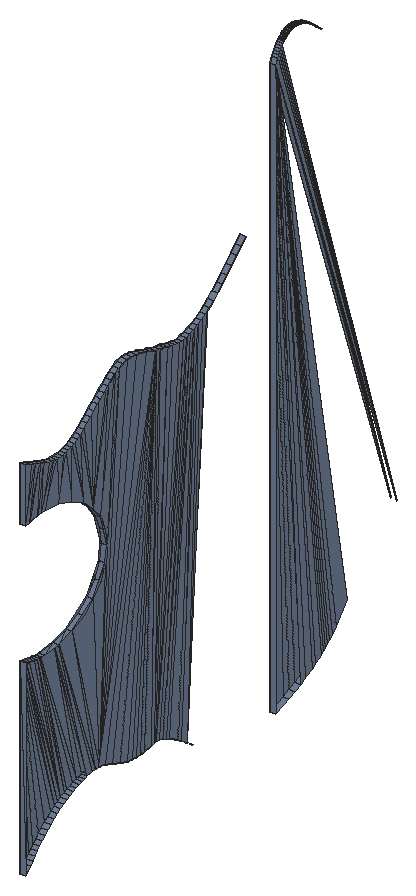
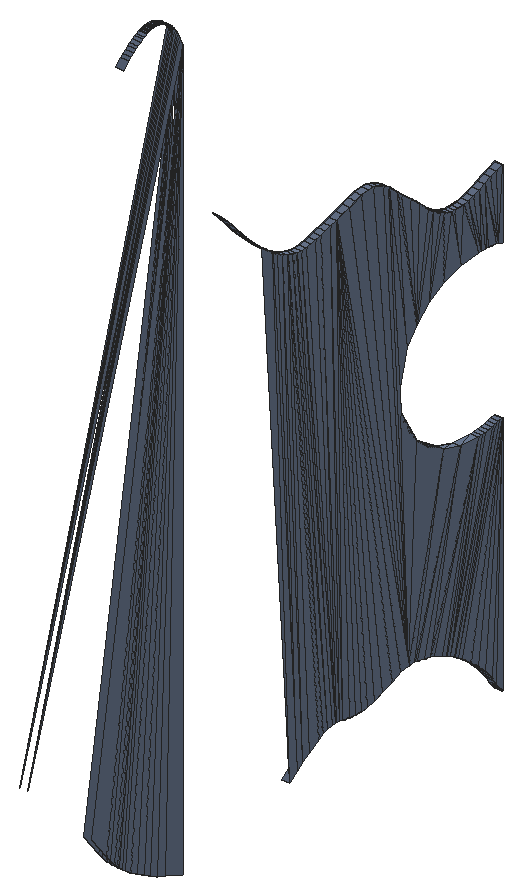
# SketchUp Ruby script. Lengths in inches.
U = 1.inch
M = Sketchup.active_model
def pt(a) = Geom::Point3d.new(a.map { |v| v * U })
def face(e, loops, mat)
  f = e.add_face(loops[0].map { |a| pt(a) })
  loops[1..].each { |l| e.add_face(l.map { |a| pt(a) }).erase! }
  f.material = f.back_material = mat if mat
  f
end
# faces: each face lists its corners as indices into pts; further lists are holes
def faces(e, pts, list, mat = nil) = list.each { |f| face(e, (f[0].is_a?(Array) ? f : [f]).map { |l| l.map { |i| pts[i] } }, mat) }
# xy, xz, yz: faces in a plane at the given z, y or x. An outline is a flat list of corners, or four numbers for a rectangle; further outlines are holes
def ring(l) = l.size == 4 ? [[l[0], l[1]], [l[2], l[1]], [l[2], l[3]], [l[0], l[3]]] : l.each_slice(2).to_a
def flat(e, list, mat, &to3) = list.each { |f| face(e, (f[0].is_a?(Array) ? f : [f]).map { |l| ring(l).map { |u, v| to3.(u, v) } }, mat) }
def xy(e, z, list, mat = nil) = flat(e, list, mat) { |x, y| [x, y, z] }
def xz(e, y, list, mat = nil) = flat(e, list, mat) { |x, z| [x, y, z] }
def yz(e, x, list, mat = nil) = flat(e, list, mat) { |y, z| [x, y, z] }
def lines(e, pts, list) = list.each { |a, b| e.add_line(pt(pts[a]), pt(pts[b])) }
# prism: a flat outline (further loops are holes) pulled along v
def prism(e, loops, v, mat = nil)
  f = face(e, loops, mat); d = Geom::Vector3d.new(v.map { |x| x * U })
  f.pushpull(f.normal.samedirection?(d) ? d.length : -d.length)
end
def box(e, o, s, mat = nil) = prism(e, [[o, [o[0] + s[0], o[1], o[2]], [o[0] + s[0], o[1] + s[1], o[2]], [o[0], o[1] + s[1], o[2]]]], [0, 0, s[2]], mat)
def at(x, y, z, deg = 0) = Geom::Transformation.translation(pt([x, y, z])) * Geom::Transformation.rotation(ORIGIN, Z_AXIS, deg.degrees)
def axes(o, x, y, z) = Geom::Transformation.new([*x, 0, *y, 0, *z, 0, *pt(o).to_a, 1])
def part(name) = M.definitions.add(name)
# library, detail: a bought-in or finely detailed component or shape, given as its bounding box
def library(name, o, s) = part(name).tap { |d| box(d.entities, o, s) }
def detail(e, o, s) = box(e.add_group.entities, o, s)
def put(e, d, t, mat = nil) = e.add_instance(d, t).tap { |i| i.material = mat if mat }
def group(e, t, mat = nil) = e.add_group.tap { |g| g.transformation = t; g.material = mat if mat }.entities
root = M.entities
M.materials.add("3D66_SU_1584934530605_002").color = [112, 126, 151]
xy(root,50.943,[[122.497,228.886,123.073,229.12]],"3D66_SU_1584934530605_002")
xz(root,216.339,[[122.497,46.745,123.073,46.745,122.497,64.189],[123.073,46.745,123.073,64.189,122.497,64.189],[122.497,75.394,123.073,80.381]],"3D66_SU_1584934530605_002")
xz(root,244.866,[[122.497,47.514,123.073,100.534]],"3D66_SU_1584934530605_002")
yz(root,122.497,[[216.339,46.745,216.339,64.189,216.821,47.359],[216.339,46.745,216.821,47.359,216.584,47.051],[216.821,47.359,216.339,64.189,217.294,47.975],[216.821,47.359,217.294,47.975,217.055,47.668],[244.866,47.514,244.866,100.534,246.341,48.072],
  [217.294,47.975,216.339,64.189,217.809,48.58],[217.294,47.975,217.809,48.58,217.543,48.28],[246.341,48.072,244.866,100.534,247.028,48.369],[247.028,48.369,244.866,100.534,247.682,48.677],[217.809,48.58,216.339,64.189,218.416,49.169],
  [217.809,48.58,218.416,49.169,218.099,48.874],[247.682,48.677,244.866,100.534,248.302,48.997],[248.302,48.997,244.866,100.534,248.888,49.328],[218.416,49.169,216.339,64.189,219.117,49.767],[218.416,49.169,219.117,49.767,218.758,49.469],
  [235.314,49.199,234.68,49.635,236.828,83.746],[235.314,49.199,236.828,83.746,237.763,84.427],[248.888,49.328,244.866,100.534,249.441,49.671],[234.68,49.635,234.12,50.01,235.941,83.225],[234.68,49.635,235.941,83.225,236.38,83.465],
  [234.68,49.635,236.38,83.465,236.828,83.746],[249.441,49.671,244.866,100.534,249.961,50.026],[219.117,49.767,216.339,64.189,219.858,50.331],[219.117,49.767,219.858,50.331,219.486,50.056],[234.12,50.01,233.621,50.329,235.506,83.026],
  [234.12,50.01,235.506,83.026,235.941,83.225],[249.961,50.026,244.866,100.534,250.206,50.211],[250.206,50.211,244.866,100.534,250.441,50.403],[233.621,50.329,232.746,50.819,235.506,83.026],[233.621,50.329,233.168,50.597,232.746,50.819],
  [219.858,50.331,216.339,64.189,220.227,50.584],[250.441,50.403,244.866,100.534,250.665,50.602],[220.227,50.584,216.339,64.189,216.63,64.114],[220.227,50.584,216.63,64.114,220.586,50.809],[250.665,50.602,244.866,100.534,250.879,50.807],
  [250.879,50.807,244.866,100.534,251.28,51.228],[220.586,50.809,216.63,64.114,216.925,64.049],[220.586,50.809,216.925,64.049,220.939,51.006],[232.746,50.819,232.342,50.998,235.506,83.026],[228.886,50.943,228.408,50.975,231.095,83.28],
  [228.886,50.943,228.653,50.952,228.408,50.975],[228.886,50.943,229.369,50.948,229.12,50.943],[228.886,50.943,231.095,83.28,229.369,50.948],[229.369,50.948,229.9375,50.983,229.644,50.954],[229.369,50.948,231.095,83.28,229.9375,50.983],
  [228.408,50.975,227.831,51.075,231.095,83.28],[228.408,50.975,228.139,51.014,227.831,51.075],[229.9375,50.983,230.538,51.124,230.234,51.047],[229.9375,50.983,231.095,83.28,230.538,51.124],[232.342,50.998,231.94,51.141,235.072,82.87],
  [232.342,50.998,235.072,82.87,235.506,83.026],[220.939,51.006,216.925,64.049,217.225,63.994],[220.939,51.006,217.225,63.994,217.84,63.919],[220.939,51.006,217.84,63.919,218.154,63.9],[220.939,51.006,218.154,63.9,221.296,51.182],
  [227.831,51.075,227.076,51.307,231.095,83.28],[227.831,51.075,227.474,51.172,227.076,51.307],[230.538,51.124,231.095,83.28,231.606,83.16],[230.538,51.124,231.606,83.16,230.856,51.193],[231.94,51.141,231.552,51.223,234.635,82.758],
  [231.94,51.141,234.635,82.758,235.072,82.87],[221.296,51.182,218.154,63.9,218.472,63.893],[221.296,51.182,218.472,63.893,221.652,51.338],[230.856,51.193,231.606,83.16,232.525,82.954],[230.856,51.193,232.525,82.954,231.192,51.233],
  [231.552,51.223,231.192,51.233,234.204,82.703],[231.552,51.223,234.204,82.703,234.635,82.758],[251.28,51.228,244.866,100.534,251.649,51.658],[231.192,51.233,232.525,82.954,232.954,82.85],[231.192,51.233,232.954,82.85,233.785,82.709],
  [231.192,51.233,233.785,82.709,234.204,82.703],[227.076,51.307,226.217,51.624,231.095,83.28],[227.076,51.307,226.651,51.463,226.217,51.624],[221.652,51.338,218.472,63.893,222.351,51.595],[221.652,51.338,222.351,51.595,222.005,51.475],
  [222.351,51.595,218.472,63.893,222.688,51.7],[226.217,51.624,225.382,51.896,231.095,83.28],[226.217,51.624,225.789,51.774,225.382,51.896],[251.649,51.658,244.866,100.534,252.909,53.283],[222.688,51.7,218.472,63.893,220.094,64.049],
  [222.688,51.7,220.094,64.049,223.313,51.868],[222.688,51.7,223.313,51.868,223.012,51.79],[223.313,51.868,220.094,64.049,223.857,51.982],[223.313,51.868,223.857,51.982,223.591,51.932],[225.382,51.896,224.689,52.012,231.095,83.28],
  [225.382,51.896,225.014,51.975,224.689,52.012],[223.857,51.982,220.094,64.049,224.121,52.013],[224.689,52.012,221.584,64.493,223.994,66.104],[224.689,52.012,224.121,52.013,221.584,64.493],[224.689,52.012,223.994,66.104,225.363,68.44],
  [224.689,52.012,224.395,52.024,224.121,52.013],[224.689,52.012,225.363,68.44,226.474,83.368],[224.689,52.012,226.474,83.368,226.892,83.643],[224.689,52.012,226.892,83.643,227.796,83.981],[224.689,52.012,227.796,83.981,228.841,83.933],
  [224.689,52.012,228.841,83.933,229.98,83.626],[224.689,52.012,229.98,83.626,231.095,83.28],[224.121,52.013,220.094,64.049,221.584,64.493],[258.624,58.923,244.866,100.534,245.073,101.017],[258.624,58.923,245.073,101.017,245.182,101.236],
  [258.624,58.923,245.182,101.236,245.295,101.441],[258.624,58.923,245.295,101.441,245.412,101.631],[258.624,58.923,245.412,101.631,245.534,101.806],[258.624,58.923,245.534,101.806,245.659,101.967],[217.84,63.919,217.225,63.994,217.53,63.951],
  [221.584,64.493,222.898,65.19,223.994,66.104],[223.994,66.104,224.83,67.199,225.363,68.44],[225.363,68.44,225.55,69.792,226.474,83.368],[225.55,69.792,224.83,72.384,226.474,83.368],[225.55,69.792,225.363,71.143,224.83,72.384],
  [224.83,72.384,223.994,73.48,225.675,82.718],[224.83,72.384,225.675,82.718,226.474,83.368],[223.994,73.48,222.581,80.149,222.953,80.431],[223.994,73.48,222.898,74.393,222.581,80.149],[223.994,73.48,222.953,80.431,223.712,81.089],
  [223.994,73.48,223.712,81.089,224.491,81.767],[223.994,73.48,224.491,81.767,225.283,82.385],[223.994,73.48,225.283,82.385,225.675,82.718],[222.898,74.393,221.538,79.578,221.866,79.734],[222.898,74.393,221.584,75.09,221.538,79.578],
  [222.898,74.393,221.866,79.734,222.581,80.149],[221.584,75.09,220.094,75.534,220.899,79.359],[221.584,75.09,220.899,79.359,221.538,79.578],[216.339,75.394,216.339,80.381,216.63,75.469],[216.63,75.469,216.339,80.381,216.844,80.21],
  [216.63,75.469,216.844,80.21,217.361,80.019],[216.63,75.469,217.361,80.019,217.881,79.823],[216.63,75.469,217.881,79.823,216.925,75.535],[220.094,75.534,218.472,75.69,219.806,79.29],[220.094,75.534,219.806,79.29,220.564,79.3],
  [220.094,75.534,220.564,79.3,220.899,79.359],[216.925,75.535,217.53,75.633,217.225,75.589],[216.925,75.535,217.881,79.823,217.53,75.633],[217.53,75.633,217.881,79.823,217.84,75.664],[217.84,75.664,217.881,79.823,218.394,79.637],
  [217.84,75.664,218.394,79.637,218.154,75.683],[218.154,75.683,218.394,79.637,218.893,79.477],[218.154,75.683,218.893,79.477,219.366,79.356],[218.154,75.683,219.366,79.356,218.472,75.69],[218.472,75.69,219.366,79.356,219.806,79.29],
  [220.203,79.277,220.564,79.3,219.806,79.29],[220.899,79.359,221.22,79.453,221.538,79.578],[221.866,79.734,222.215,79.919,222.581,80.149],[222.953,80.431,223.33,80.749,223.712,81.089],[223.712,81.089,224.099,81.433,224.491,81.767],
  [224.491,81.767,224.888,82.075,225.283,82.385],[233.785,82.709,232.954,82.85,233.371,82.763],[225.675,82.718,226.07,83.053,226.474,83.368],[232.525,82.954,231.606,83.16,232.079,83.063],[231.095,83.28,229.98,83.626,230.548,83.444],
  [229.98,83.626,228.841,83.933,229.406,83.798],[226.892,83.643,227.331,83.854,227.796,83.981],[236.828,83.746,237.287,84.067,237.763,84.427],[228.841,83.933,227.796,83.981,228.299,84.003],[238.258,84.844,238.77,85.324,239.294,85.85],
  [239.294,85.85,239.827,86.405,240.362,86.971],[240.362,86.971,240.896,87.532,241.424,88.069]],"3D66_SU_1584934530605_002")
yz(root,123.073,[[247.682,48.677,248.302,48.997,244.866,100.534],[248.302,48.997,248.888,49.328,244.866,100.534],[248.888,49.328,249.441,49.671,244.866,100.534],[234.68,49.635,235.941,83.225,234.12,50.01],[234.68,49.635,236.38,83.465,235.941,83.225],
  [234.68,49.635,236.828,83.746,236.38,83.465],[249.441,49.671,249.961,50.026,244.866,100.534],[234.12,50.01,235.506,83.026,233.621,50.329],[234.12,50.01,235.941,83.225,235.506,83.026],[249.961,50.026,250.206,50.211,244.866,100.534],
  [250.206,50.211,250.441,50.403,244.866,100.534],[233.621,50.329,232.746,50.819,233.168,50.597],[233.621,50.329,235.506,83.026,232.746,50.819],[250.441,50.403,250.665,50.602,244.866,100.534],[250.665,50.602,250.879,50.807,244.866,100.534],
  [250.879,50.807,251.28,51.228,244.866,100.534],[232.746,50.819,235.506,83.026,232.342,50.998],[228.886,50.943,228.408,50.975,228.653,50.952],[228.886,50.943,231.095,83.28,228.408,50.975],[228.886,50.943,229.12,50.943,229.369,50.948],
  [228.886,50.943,229.369,50.948,231.095,83.28],[229.369,50.948,229.644,50.954,229.9375,50.983],[229.369,50.948,229.9375,50.983,231.095,83.28],[228.408,50.975,227.831,51.075,228.139,51.014],[228.408,50.975,231.095,83.28,227.831,51.075],
  [229.9375,50.983,230.234,51.047,230.538,51.124],[229.9375,50.983,230.538,51.124,231.095,83.28],[232.342,50.998,235.072,82.87,231.94,51.141],[232.342,50.998,235.506,83.026,235.072,82.87],[227.831,51.075,227.076,51.307,227.474,51.172],
  [227.831,51.075,231.095,83.28,227.076,51.307],[230.538,51.124,230.856,51.193,231.606,83.16],[230.538,51.124,231.606,83.16,231.095,83.28],[231.94,51.141,234.635,82.758,231.552,51.223],[231.94,51.141,235.072,82.87,234.635,82.758],
  [230.856,51.193,231.192,51.233,232.525,82.954],[230.856,51.193,232.525,82.954,231.606,83.16],[231.552,51.223,234.204,82.703,231.192,51.233],[231.552,51.223,234.635,82.758,234.204,82.703],[251.28,51.228,251.649,51.658,244.866,100.534],
  [231.192,51.233,232.954,82.85,232.525,82.954],[231.192,51.233,233.785,82.709,232.954,82.85],[231.192,51.233,234.204,82.703,233.785,82.709],[227.076,51.307,226.217,51.624,226.651,51.463],[227.076,51.307,231.095,83.28,226.217,51.624],
  [226.217,51.624,225.382,51.896,225.789,51.774],[226.217,51.624,231.095,83.28,225.382,51.896],[251.649,51.658,252.909,53.283,244.866,100.534],[223.313,51.868,223.857,51.982,220.094,64.049],[223.313,51.868,223.591,51.932,223.857,51.982],
  [225.382,51.896,224.689,52.012,225.014,51.975],[225.382,51.896,231.095,83.28,224.689,52.012],[223.857,51.982,224.121,52.013,220.094,64.049],[224.689,52.012,221.584,64.493,224.121,52.013],[224.689,52.012,223.994,66.104,221.584,64.493],
  [224.689,52.012,225.363,68.44,223.994,66.104],[224.689,52.012,224.121,52.013,224.395,52.024],[224.689,52.012,225.55,69.792,225.363,68.44],[224.689,52.012,226.892,83.643,225.55,69.792],[224.689,52.012,227.796,83.981,226.892,83.643],
  [224.689,52.012,228.841,83.933,227.796,83.981],[224.689,52.012,229.98,83.626,228.841,83.933],[224.689,52.012,231.095,83.28,229.98,83.626],[224.121,52.013,221.584,64.493,220.094,64.049],[258.624,58.923,245.073,101.017,244.866,100.534],
  [258.624,58.923,245.182,101.236,245.073,101.017],[258.624,58.923,245.295,101.441,245.182,101.236],[258.624,58.923,245.412,101.631,245.295,101.441],[258.624,58.923,245.534,101.806,245.412,101.631],[221.584,64.493,223.994,66.104,222.898,65.19],
  [223.994,66.104,225.363,68.44,224.83,67.199],[225.55,69.792,224.83,72.384,225.363,71.143],[225.55,69.792,226.474,83.368,224.83,72.384],[225.55,69.792,226.892,83.643,226.474,83.368],[224.83,72.384,225.675,82.718,223.994,73.48],
  [224.83,72.384,226.474,83.368,225.675,82.718],[223.994,73.48,222.581,80.149,222.898,74.393],[223.994,73.48,222.953,80.431,222.581,80.149],[223.994,73.48,223.712,81.089,222.953,80.431],[223.994,73.48,224.491,81.767,223.712,81.089],
  [223.994,73.48,225.283,82.385,224.491,81.767],[223.994,73.48,225.675,82.718,225.283,82.385],[222.898,74.393,221.538,79.578,221.584,75.09],[222.898,74.393,221.866,79.734,221.538,79.578],[222.898,74.393,222.581,80.149,221.866,79.734],
  [221.584,75.09,220.899,79.359,220.094,75.534],[221.584,75.09,221.538,79.578,220.899,79.359],[216.339,75.394,216.63,75.469,217.361,80.019],[216.339,75.394,216.844,80.21,216.339,80.381],[216.339,75.394,217.361,80.019,216.844,80.21],
  [216.63,75.469,216.925,75.535,217.881,79.823],[216.63,75.469,217.881,79.823,217.361,80.019],[220.094,75.534,219.806,79.29,218.472,75.69],[220.094,75.534,220.564,79.3,219.806,79.29],[220.094,75.534,220.899,79.359,220.564,79.3],
  [216.925,75.535,217.225,75.589,217.53,75.633],[216.925,75.535,217.53,75.633,217.881,79.823],[217.53,75.633,217.84,75.664,217.881,79.823],[217.84,75.664,218.154,75.683,218.394,79.637],[217.84,75.664,218.394,79.637,217.881,79.823],
  [218.154,75.683,218.472,75.69,219.366,79.356],[218.154,75.683,218.893,79.477,218.394,79.637],[218.154,75.683,219.366,79.356,218.893,79.477],[218.472,75.69,219.806,79.29,219.366,79.356],[220.203,79.277,219.806,79.29,220.564,79.3],
  [220.899,79.359,221.538,79.578,221.22,79.453],[221.866,79.734,222.581,80.149,222.215,79.919],[222.953,80.431,223.712,81.089,223.33,80.749],[223.712,81.089,224.491,81.767,224.099,81.433],[224.491,81.767,225.283,82.385,224.888,82.075],
  [233.785,82.709,233.371,82.763,232.954,82.85],[225.675,82.718,226.474,83.368,226.07,83.053],[232.525,82.954,232.079,83.063,231.606,83.16],[231.095,83.28,230.548,83.444,229.98,83.626],[229.98,83.626,229.406,83.798,228.841,83.933],
  [226.892,83.643,227.796,83.981,227.331,83.854],[236.828,83.746,237.763,84.427,237.287,84.067],[228.841,83.933,228.299,84.003,227.796,83.981],[238.258,84.844,239.294,85.85,238.77,85.324],[239.294,85.85,240.362,86.971,239.827,86.405],
  [240.362,86.971,241.424,88.069,240.896,87.532]],"3D66_SU_1584934530605_002")
p = [[123.073,216.584,47.051],[123.073,216.339,46.745],[122.497,216.339,46.745],[122.497,216.584,47.051],[122.497,216.821,47.359],[123.073,216.821,47.359],
  [122.497,217.055,47.668],[123.073,217.055,47.668],[123.073,244.866,47.514],[122.497,244.866,47.514],[122.497,246.341,48.072],[123.073,246.341,48.072],
  [122.497,217.294,47.975],[123.073,217.294,47.975],[122.497,217.543,48.28],[123.073,217.543,48.28],[122.497,247.028,48.369],[123.073,247.028,48.369],
  [122.497,217.809,48.58],[123.073,217.809,48.58],[122.497,247.682,48.677],[123.073,247.682,48.677],[122.497,218.099,48.874],[123.073,218.099,48.874],
  [122.497,248.302,48.997],[123.073,248.302,48.997],[122.497,218.416,49.169],[123.073,218.416,49.169],[122.497,248.888,49.328],[123.073,248.888,49.328],
  [122.497,218.758,49.469],[123.073,218.758,49.469],[122.497,235.314,49.199],[123.073,235.314,49.199],[123.073,234.68,49.635],[122.497,234.68,49.635],
  [122.497,249.441,49.671],[123.073,249.441,49.671],[122.497,219.117,49.767],[123.073,219.117,49.767],[123.073,234.12,50.01],[122.497,234.12,50.01],
  [122.497,249.961,50.026],[123.073,249.961,50.026],[122.497,219.486,50.056],[123.073,219.486,50.056],[123.073,233.621,50.329],[122.497,233.621,50.329],
  [122.497,219.858,50.331],[123.073,219.858,50.331],[122.497,220.227,50.584],[123.073,220.227,50.584],[123.073,233.168,50.597],[122.497,233.168,50.597],
  [122.497,220.586,50.809],[123.073,220.586,50.809],[123.073,232.746,50.819],[122.497,232.746,50.819],[122.497,220.939,51.006],[123.073,220.939,51.006],
  [123.073,232.342,50.998],[122.497,232.342,50.998],[122.497,228.886,50.943],[123.073,228.886,50.943],[123.073,228.653,50.952],[122.497,228.653,50.952],
  [122.497,229.369,50.948],[123.073,229.369,50.948],[123.073,229.12,50.943],[122.497,229.12,50.943],[122.497,229.644,50.954],[123.073,229.644,50.954],
  [122.497,221.296,51.182],[123.073,221.296,51.182],[122.497,228.139,51.014],[123.073,228.139,51.014],[123.073,227.831,51.075],[122.497,227.831,51.075],
  [122.497,228.408,50.975],[123.073,228.408,50.975],[122.497,229.9375,50.983],[123.073,229.9375,50.983],[122.497,230.234,51.047],[123.073,230.234,51.047],
  [123.073,230.538,51.124],[122.497,230.538,51.124],[123.073,231.94,51.141],[122.497,231.94,51.141],[123.073,227.474,51.172],[122.497,227.474,51.172],
  [122.497,230.856,51.193],[123.073,230.856,51.193],[123.073,231.552,51.223],[122.497,231.552,51.223],[122.497,221.652,51.338],[123.073,221.652,51.338],
  [123.073,227.076,51.307],[122.497,227.076,51.307],[122.497,231.192,51.233],[123.073,231.192,51.233],[122.497,222.005,51.475],[123.073,222.005,51.475],
  [123.073,226.651,51.463],[122.497,226.651,51.463],[122.497,222.351,51.595],[123.073,222.351,51.595],[123.073,226.217,51.624],[122.497,226.217,51.624],
  [122.497,222.688,51.7],[123.073,222.688,51.7],[123.073,225.789,51.774],[122.497,225.789,51.774],[122.497,223.012,51.79],[123.073,223.012,51.79],
  [122.497,223.313,51.868],[123.073,223.313,51.868],[123.073,225.382,51.896],[122.497,225.382,51.896],[122.497,223.591,51.932],[123.073,223.591,51.932],
  [122.497,223.857,51.982],[123.073,223.857,51.982],[123.073,225.014,51.975],[122.497,225.014,51.975],[122.497,224.121,52.013],[123.073,224.121,52.013],
  [122.497,224.395,52.024],[123.073,224.395,52.024],[122.497,224.689,52.012],[123.073,224.689,52.012],[122.497,217.53,63.951],[123.073,217.53,63.951],
  [123.073,217.84,63.919],[122.497,217.84,63.919],[123.073,218.154,63.9],[122.497,218.154,63.9],[123.073,218.472,63.893],[122.497,218.472,63.893],
  [122.497,220.094,64.049],[123.073,220.094,64.049],[122.497,216.63,64.114],[123.073,216.63,64.114],[123.073,216.925,64.049],[122.497,216.925,64.049],
  [123.073,217.225,63.994],[122.497,217.225,63.994],[122.497,221.584,64.493],[123.073,221.584,64.493],[122.497,216.339,64.189],[123.073,216.339,64.189],
  [123.073,222.898,65.19],[122.497,222.898,65.19],[123.073,223.994,66.104],[122.497,223.994,66.104],[123.073,224.83,67.199],[122.497,224.83,67.199],
  [123.073,225.363,68.44],[122.497,225.363,68.44],[123.073,225.55,69.792],[122.497,225.55,69.792],[123.073,225.363,71.143],[122.497,225.363,71.143],
  [123.073,224.83,72.384],[122.497,224.83,72.384],[123.073,223.994,73.48],[122.497,223.994,73.48],[123.073,222.898,74.393],[122.497,222.898,74.393],
  [123.073,221.584,75.09],[122.497,221.584,75.09],[123.073,220.094,75.534],[122.497,220.094,75.534],[122.497,216.63,75.469],[123.073,216.63,75.469],
  [123.073,216.339,75.394],[122.497,216.339,75.394],[122.497,216.925,75.535],[123.073,216.925,75.535],[122.497,217.225,75.589],[123.073,217.225,75.589],
  [123.073,218.472,75.69],[122.497,218.472,75.69],[122.497,217.53,75.633],[123.073,217.53,75.633],[122.497,217.84,75.664],[123.073,217.84,75.664],
  [122.497,218.154,75.683],[123.073,218.154,75.683],[122.497,219.366,79.356],[123.073,219.366,79.356],[123.073,219.806,79.29],[122.497,219.806,79.29],
  [123.073,220.203,79.277],[122.497,220.203,79.277],[123.073,220.564,79.3],[122.497,220.564,79.3],[123.073,220.899,79.359],[122.497,220.899,79.359],
  [122.497,218.893,79.477],[123.073,218.893,79.477],[123.073,221.22,79.453],[122.497,221.22,79.453],[122.497,218.394,79.637],[123.073,218.394,79.637],
  [123.073,221.538,79.578],[122.497,221.538,79.578],[122.497,217.881,79.823],[123.073,217.881,79.823],[123.073,221.866,79.734],[122.497,221.866,79.734],
  [123.073,222.215,79.919],[122.497,222.215,79.919],[122.497,217.361,80.019],[123.073,217.361,80.019],[123.073,222.581,80.149],[122.497,222.581,80.149],
  [122.497,216.844,80.21],[123.073,216.844,80.21],[123.073,222.953,80.431],[122.497,222.953,80.431],[122.497,216.339,80.381],[123.073,216.339,80.381],
  [123.073,223.33,80.749],[122.497,223.33,80.749],[123.073,223.712,81.089],[122.497,223.712,81.089],[123.073,224.099,81.433],[122.497,224.099,81.433],
  [123.073,224.491,81.767],[122.497,224.491,81.767],[123.073,224.888,82.075],[122.497,224.888,82.075],[123.073,225.283,82.385],[122.497,225.283,82.385],
  [123.073,225.675,82.718],[122.497,225.675,82.718],[123.073,226.07,83.053],[122.497,226.07,83.053],[122.497,233.371,82.763],[123.073,233.371,82.763],
  [123.073,233.785,82.709],[122.497,233.785,82.709],[123.073,234.204,82.703],[122.497,234.204,82.703],[123.073,234.635,82.758],[122.497,234.635,82.758],
  [122.497,232.525,82.954],[123.073,232.525,82.954],[123.073,232.954,82.85],[122.497,232.954,82.85],[123.073,235.072,82.87],[122.497,235.072,82.87],
  [123.073,235.506,83.026],[122.497,235.506,83.026],[122.497,232.079,83.063],[123.073,232.079,83.063],[123.073,235.941,83.225],[122.497,235.941,83.225],
  [123.073,226.474,83.368],[122.497,226.474,83.368],[122.497,231.606,83.16],[123.073,231.606,83.16],[122.497,231.095,83.28],[123.073,231.095,83.28],
  [123.073,236.38,83.465],[122.497,236.38,83.465],[122.497,230.548,83.444],[123.073,230.548,83.444],[123.073,226.892,83.643],[122.497,226.892,83.643],
  [122.497,229.98,83.626],[123.073,229.98,83.626],[123.073,236.828,83.746],[122.497,236.828,83.746],[123.073,227.331,83.854],[122.497,227.331,83.854],
  [122.497,229.406,83.798],[123.073,229.406,83.798],[123.073,237.287,84.067],[122.497,237.287,84.067],[122.497,228.841,83.933],[123.073,228.841,83.933],
  [123.073,227.796,83.981],[122.497,227.796,83.981],[122.497,228.299,84.003],[123.073,228.299,84.003],[123.073,237.763,84.427],[122.497,237.763,84.427],
  [123.073,238.258,84.844],[122.497,238.258,84.844],[123.073,238.77,85.324],[122.497,238.77,85.324],[123.073,239.294,85.85],[122.497,239.294,85.85],
  [123.073,239.827,86.405],[122.497,239.827,86.405],[123.073,240.362,86.971],[122.497,240.362,86.971],[123.073,240.896,87.532],[122.497,240.896,87.532],
  [123.073,241.424,88.069],[122.497,241.424,88.069],[123.073,245.073,101.017],[122.497,245.073,101.017],[122.497,244.866,100.534],[123.073,244.866,100.534],
  [123.073,245.182,101.236],[122.497,245.182,101.236],[123.073,245.295,101.441],[122.497,245.295,101.441],[123.073,250.098,101.214],[122.497,250.098,101.214],
  [122.497,249.666,101.613],[123.073,249.666,101.613],[123.073,245.412,101.631],[122.497,245.412,101.631],[123.073,245.534,101.806],[122.497,245.534,101.806],
  [122.497,249.453,101.791],[123.073,249.453,101.791],[123.073,245.659,101.967],[122.497,245.659,101.967],[122.497,249.242,101.954],[123.073,249.242,101.954],
  [123.073,245.788,102.113],[122.497,245.788,102.113],[122.497,249.034,102.101],[123.073,249.034,102.101],[122.497,245.855,102.181],[123.073,245.855,102.181],
  [122.497,248.828,102.234],[123.073,248.828,102.234],[123.073,245.922,102.245],[122.497,245.922,102.245],[122.497,245.99,102.305],[123.073,245.99,102.305],
  [122.497,248.625,102.352],[123.073,248.625,102.352],[122.497,246.059,102.361],[123.073,246.059,102.361],[122.497,246.129,102.414],[123.073,246.129,102.414],
  [122.497,246.201,102.463],[123.073,246.201,102.463],[122.497,248.425,102.456],[123.073,248.425,102.456],[122.497,246.273,102.509],[123.073,246.273,102.509],
  [122.497,246.346,102.551],[123.073,246.346,102.551],[123.073,248.229,102.544],[122.497,248.229,102.544],[122.497,248.036,102.618],[123.073,248.036,102.618],
  [123.073,246.42,102.589],[122.497,246.42,102.589],[123.073,246.496,102.623],[122.497,246.496,102.623],[123.073,246.572,102.654],[122.497,246.572,102.654],
  [123.073,247.941,102.649],[122.497,247.941,102.649],[122.497,247.847,102.677],[123.073,247.847,102.677],[123.073,246.649,102.681],[122.497,246.649,102.681],
  [123.073,246.727,102.705],[122.497,246.727,102.705],[123.073,246.806,102.725],[122.497,246.806,102.725],[123.073,246.887,102.741],[122.497,246.887,102.741],
  [123.073,246.968,102.753],[122.497,246.968,102.753],[123.073,247.571,102.738],[122.497,247.571,102.738],[122.497,247.481,102.751],[123.073,247.481,102.751],
  [123.073,247.662,102.722],[122.497,247.662,102.722],[123.073,247.754,102.701],[122.497,247.754,102.701],[123.073,247.05,102.762],[122.497,247.05,102.762],
  [123.073,247.134,102.767],[122.497,247.134,102.767],[123.073,247.219,102.769],[122.497,247.219,102.769],[123.073,247.305,102.767],[122.497,247.305,102.767],
  [123.073,247.393,102.761],[122.497,247.393,102.761]]
faces(root,p,[[0,1,2],[0,2,3],[4,5,0,3],[6,7,5,4],[8,9,10,11],[12,13,7,6],[14,15,13,12],[11,10,16,17],
  [18,19,15,14],[17,16,20,21],[22,23,19,18],[21,20,24,25],[26,27,23,22],[25,24,28,29],[30,31,27,26],[32,33,34,35],
  [29,28,36,37],[38,39,31,30],[35,34,40,41],[37,36,42,43],[44,45,39,38],[41,40,46,47],[48,49,45,44],[50,51,49,48],
  [47,46,52,53],[54,55,51,50],[53,52,56,57],[58,59,55,54],[57,56,60,61],[62,63,64,65],[66,67,68,69],[70,71,67,66],
  [72,73,59,58],[74,75,76,77],[78,79,75,74],[65,64,79,78],[80,81,71,70],[82,83,81,80],[84,83,82],[84,82,85],
  [61,60,86,87],[77,76,88,89],[90,91,84,85],[87,86,92,93],[94,95,73,72],[89,88,96,97],[98,99,91,90],[93,92,99,98],
  [100,101,95,94],[97,96,102,103],[104,105,101,100],[103,102,106,107],[108,109,105,104],[107,106,110,111],[112,113,109,108],[114,115,113,112],
  [111,110,116,117],[118,119,115,114],[120,121,119,118],[117,116,122,123],[124,125,121,120],[126,127,125,124],[128,129,127,126],[123,122,129,128],
  [130,131,132,133],[133,132,134,135],[135,134,136,137],[136,138,137],[136,139,138],[140,141,142,143],[143,142,144,145],[145,144,131,130],
  [139,146,138],[139,147,146],[148,149,141,140],[146,147,150,151],[151,150,152,153],[153,152,154,155],[155,154,156,157],[157,156,158,159],
  [159,158,160,161],[161,160,162,163],[163,162,164,165],[165,164,166,167],[167,166,168,169],[169,168,170,171],[172,173,174,175],[176,177,173,172],
  [178,179,177,176],[171,170,180,181],[182,183,179,178],[184,185,183,182],[186,187,185,184],[181,180,187,186],[188,189,190,191],[191,190,192,193],
  [193,192,194,195],[195,194,196,197],[198,199,189,188],[197,196,200,201],[202,203,199,198],[201,200,204,205],[206,207,203,202],[205,204,208,209],
  [209,208,210,211],[212,213,207,206],[211,210,214,215],[216,217,213,212],[215,214,218,219],[220,221,217,216],[219,218,222,223],[223,222,224,225],
  [225,224,226,227],[227,226,228,229],[229,228,230,231],[231,230,232,233],[233,232,234,235],[235,234,236,237],[238,239,240,241],[241,240,242,243],
  [243,242,244,245],[246,247,248,249],[249,248,239,238],[245,244,250,251],[251,250,252,253],[254,255,247,246],[253,252,256,257],[237,236,258,259],
  [260,261,255,254],[262,263,261,260],[257,256,264,265],[266,267,263,262],[259,258,268,269],[270,271,267,266],[265,264,272,273],[269,268,274,275],
  [276,277,271,270],[273,272,278,279],[280,281,277,276],[275,274,282,283],[284,285,281,280],[283,282,285,284],[279,278,286,287],[287,286,288,289],
  [289,288,290,291],[291,290,292,293],[293,292,294,295],[295,294,296,297],[297,296,298,299],[299,298,300,301],[302,303,304,305],[306,307,303,302],
  [308,309,307,306],[310,311,312,313],[314,315,309,308],[316,317,315,314],[313,312,318,319],[320,321,317,316],[319,318,322,323],[324,325,321,320],
  [323,322,326,327],[328,325,324],[328,324,329],[327,326,330,331],[332,333,328,329],[334,333,332],[334,332,335],[331,330,336,337],
  [338,334,335],[338,335,339],[340,338,339],[340,339,341],[342,340,341],[342,341,343],[337,336,344,345],[346,342,343],
  [346,343,347],[348,346,347],[348,347,349],[350,351,352,353],[345,344,351,350],[354,355,348,349],[356,357,355,354],[358,359,357,356],
  [360,361,362,363],[353,352,361,360],[364,365,359,358],[366,367,365,364],[368,369,367,366],[370,371,369,368],[372,373,371,370],[374,375,376,377],
  [378,379,375,374],[380,381,379,378],[363,362,381,380],[382,383,373,372],[384,385,383,382],[386,387,385,384],[388,389,387,386],[390,391,389,388],
  [377,376,391,390]],"3D66_SU_1584934530605_002")
